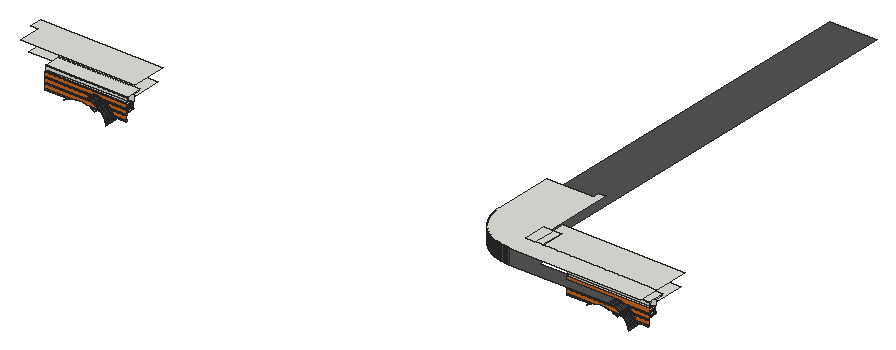
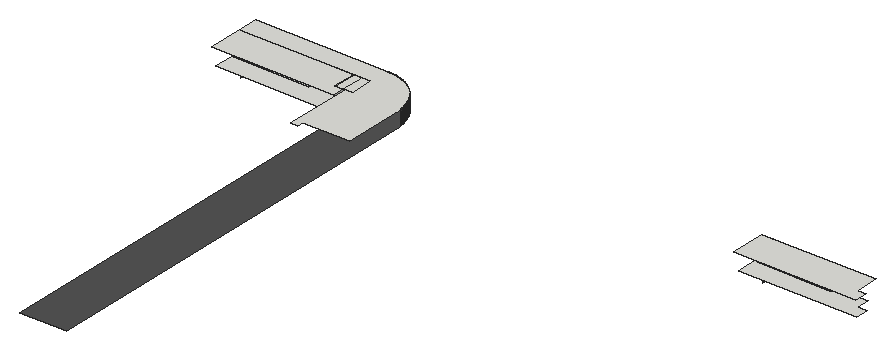
# SketchUp Ruby script. Lengths in inches.
U = 1.inch
M = Sketchup.active_model
def pt(a) = Geom::Point3d.new(a.map { |v| v * U })
def face(e, loops, mat)
  f = e.add_face(loops[0].map { |a| pt(a) })
  loops[1..].each { |l| e.add_face(l.map { |a| pt(a) }).erase! }
  f.material = f.back_material = mat if mat
  f
end
# faces: each face lists its corners as indices into pts; further lists are holes
def faces(e, pts, list, mat = nil) = list.each { |f| face(e, (f[0].is_a?(Array) ? f : [f]).map { |l| l.map { |i| pts[i] } }, mat) }
# xy, xz, yz: faces in a plane at the given z, y or x. An outline is a flat list of corners, or four numbers for a rectangle; further outlines are holes
def ring(l) = l.size == 4 ? [[l[0], l[1]], [l[2], l[1]], [l[2], l[3]], [l[0], l[3]]] : l.each_slice(2).to_a
def flat(e, list, mat, &to3) = list.each { |f| face(e, (f[0].is_a?(Array) ? f : [f]).map { |l| ring(l).map { |u, v| to3.(u, v) } }, mat) }
def xy(e, z, list, mat = nil) = flat(e, list, mat) { |x, y| [x, y, z] }
def xz(e, y, list, mat = nil) = flat(e, list, mat) { |x, z| [x, y, z] }
def yz(e, x, list, mat = nil) = flat(e, list, mat) { |y, z| [x, y, z] }
def lines(e, pts, list) = list.each { |a, b| e.add_line(pt(pts[a]), pt(pts[b])) }
# prism: a flat outline (further loops are holes) pulled along v
def prism(e, loops, v, mat = nil)
  f = face(e, loops, mat); d = Geom::Vector3d.new(v.map { |x| x * U })
  f.pushpull(f.normal.samedirection?(d) ? d.length : -d.length)
end
def box(e, o, s, mat = nil) = prism(e, [[o, [o[0] + s[0], o[1], o[2]], [o[0] + s[0], o[1] + s[1], o[2]], [o[0], o[1] + s[1], o[2]]]], [0, 0, s[2]], mat)
def at(x, y, z, deg = 0) = Geom::Transformation.translation(pt([x, y, z])) * Geom::Transformation.rotation(ORIGIN, Z_AXIS, deg.degrees)
def axes(o, x, y, z) = Geom::Transformation.new([*x, 0, *y, 0, *z, 0, *pt(o).to_a, 1])
def part(name) = M.definitions.add(name)
# library, detail: a bought-in or finely detailed component or shape, given as its bounding box
def library(name, o, s) = part(name).tap { |d| box(d.entities, o, s) }
def detail(e, o, s) = box(e.add_group.entities, o, s)
def put(e, d, t, mat = nil) = e.add_instance(d, t).tap { |i| i.material = mat if mat }
def group(e, t, mat = nil) = e.add_group.tap { |g| g.transformation = t; g.material = mat if mat }.entities
root = M.entities
M.materials.add("[0041_Chocolate]").color = [210, 105, 30]
M.materials.add("[Color M06]").color = [84, 84, 84]
xy(root,385.02,[[1547.71,280.47,1577.2,281.47],[1605.02,280.47,1649.14,281.47],[2198.21,280.47,2227.7,281.47],[2255.52,280.47,2299.64,281.47]],"[0041_Chocolate]")
xy(root,386.9375,[[1547.71,280.47,1582.17,281.47],[1600.06,280.47,1649.14,281.47],[2198.21,280.47,2232.67,281.47],[2250.56,280.47,2299.64,281.47]],"[0041_Chocolate]")
xy(root,391.89,[[1547.71,280.47,1649.14,281.47],[2198.21,280.47,2299.64,281.47]],"[0041_Chocolate]")
xy(root,393.8125,[[1547.71,280.47,1649.14,281.47],[2198.21,280.47,2299.64,281.47]],"[0041_Chocolate]")
xy(root,395.26,[[1547.71,302.46,1626.96,310.27],[2198.21,302.46,2277.46,310.27]])
xy(root,398.77,[[1547.71,280.47,1649.14,281.47],[2198.21,280.47,2299.64,281.47]],"[0041_Chocolate]")
xy(root,400.6875,[[1547.71,280.47,1649.14,281.47],[2198.21,280.47,2299.64,281.47]],"[0041_Chocolate]")
xy(root,402.64,[[1547.71,300.33,1608.92,302.46],[2198.21,300.33,2259.42,302.46],[1640.52,302.46,1643.23,302.46,1643.23,337.5625,1496.21,337.5625,1496.21,321.34,1507.74,321.34,1507.74,305.58,1547.71,305.58,1547.71,312.8125,1640.52,312.8125],[1547.71,302.46,1640.52,312.8125],[2291.02,302.46,2293.73,302.46,2293.73,337.5625,2146.71,337.5625,2146.71,321.34,2158.24,321.34,2158.24,305.58,2198.21,305.58,2198.21,312.8125,2291.02,312.8125],
  [2198.21,302.46,2291.02,312.8125],[2137,305.58,2146.71,312.8125],[2146.71,305.58,2158.24,312.8125],[2137,312.8125,2146.71,321.34]])
xy(root,402.64,[[2135.95,267.75,2134.46,267.77,2132.97,267.83,2131.49,267.93,2130.01,268.0625,2128.53,268.24,2127.05,268.45,2125.59,268.7,2124.125,268.99,2122.67,269.32,2121.23,269.6875,2119.8,270.09,2118.375,270.53,2116.96,271.01,2115.57,271.53,2114.18,272.08,2112.8125,272.67,2111.46,273.29,2110.125,273.95,2108.81,274.64,2107.51,275.37,2106.23,276.13,2104.97,276.93,2103.73,277.75,2102.51,278.61,2101.32,279.51,2100.15,280.43,2099.01,281.38,2097.89,282.36,2096.79,283.37,2095.73,284.41,2094.6875,285.48,2093.68,286.57,2092.69,287.69,2091.74,288.84,2090.82,290.01,2089.93,291.2,2089.07,292.42,2088.24,293.65,2087.45,294.91,2086.6875,296.19,2085.96,297.49,2085.27,298.8125,2084.61,300.15,2083.98,301.5,2083.4,302.87,2082.84,304.25,2082.33,305.65,2081.85,307.06,2081.41,308.48,2081,309.91,2080.64,311.36,2080.31,312.81,2080.02,314.27,2079.77,315.74,2079.55,317.21,2079.375,318.69,2079.24,320.17,2079.14,321.66,2079.08,323.15,2079.07,324.64,2079.07,838.14,2137,838.14,2137,305.58,2158.24,305.58,2158.24,287.95,2198.21,287.95,2198.21,300.33,2259.42,300.33,2259.42,267.75]],"[Color M06]")
xy(root,405.64,[[1547.71,280.47,1649.14,281.47],[2198.21,280.47,2299.64,281.47]],"[0041_Chocolate]")
xy(root,411.82,[[1547.71,281.47,1649.14,302.46],[2198.21,281.47,2299.64,302.46]])
xy(root,421.25,[[2135.95,267.75,2300.52,267.75,2300.52,292.45,2137,292.45,2137,321.34,2145.53,321.34,2145.53,406.38,2137,406.38,2137,397.86,2079.07,397.86,2079.07,324.64,2079.08,323.15,2079.14,321.66,2079.24,320.17,2079.375,318.69,2079.55,317.21,2079.77,315.74,2080.02,314.27,2080.31,312.81,2080.64,311.36,2081,309.91,2081.41,308.48,2081.85,307.06,2082.33,305.65,2082.84,304.25,2083.4,302.87,2083.98,301.5,2084.61,300.15,2085.27,298.8125,2085.96,297.49,2086.6875,296.19,2087.45,294.91,2088.24,293.65,2089.07,292.42,2089.93,291.2,2090.82,290.01,2091.74,288.84,2092.69,287.69,2093.68,286.57,2094.6875,285.48,2095.73,284.41,2096.79,283.37,2097.89,282.36,2099.01,281.38,2100.15,280.43,2101.32,279.51,2102.51,278.61,2103.73,277.75,2104.97,276.93,2106.23,276.13,2107.51,275.37,2108.81,274.64,2110.125,273.95,2111.46,273.29,2112.8125,272.67,2114.18,272.08,2115.57,271.53,2116.96,271.01,2118.375,270.53,2119.8,270.09,2121.23,269.6875,2122.67,269.32,2124.125,268.99,2125.59,268.7,2127.05,268.45,2128.53,268.24,2130.01,268.0625,2131.49,267.93,2132.97,267.83,2134.46,267.77],[1507.74,292.45,1650.02,292.45,1650.02,336.27,1498.09,336.27,1498.09,321.34,1507.74,321.34],[2137,292.45,2148.59,321.34],[2148.59,292.45,2158.24,321.34],[2158.24,292.45,2300.52,292.45,2300.52,336.27,2148.59,336.27,2148.59,321.34,2158.24,321.34]])
xz(root,280.47,[[1547.71,386.9375,1582.17,386.9375,1587,388.23,1595.19,388.24,1600.06,386.9375,1649.14,386.9375,1649.14,391.89,1547.71,391.89],[2198.21,386.9375,2232.67,386.9375,2237.5,388.23,2245.69,388.24,2250.56,386.9375,2299.64,386.9375,2299.64,391.89,2198.21,391.89],[1547.71,393.8125,1649.14,398.77],[2198.21,393.8125,2299.64,398.77],[1547.71,400.6875,1649.14,405.64],
  [2198.21,400.6875,2299.64,405.64]],"[0041_Chocolate]")
xz(root,281.47,[[1547.71,405.64,1649.14,407.5625],[2198.21,405.64,2299.64,407.5625],[1547.71,407.5625,1649.14,411.82],[2198.21,407.5625,2299.64,411.82],[1547.71,411.82,1649.14,412.52],
  [2198.21,411.82,2299.64,412.52]])
xz(root,281.47,[[1547.71,385.02,1577.2,385.02,1579.1,386.11,1582.17,386.9375,1547.71,386.9375],[1605.02,385.02,1649.14,385.02,1649.14,386.9375,1600.06,386.9375,1603.1,386.125],[2198.21,385.02,2227.7,385.02,2229.6,386.11,2232.67,386.9375,2198.21,386.9375],[2255.52,385.02,2299.64,385.02,2299.64,386.9375,2250.56,386.9375,2253.6,386.125],[1547.71,391.89,1649.14,393.8125],
  [2198.21,391.89,2299.64,393.8125],[1547.71,398.77,1649.14,400.6875],[2198.21,398.77,2299.64,400.6875]],"[0041_Chocolate]")
xz(root,302.46,[[1547.71,395.26,1626.96,395.26,1626.65,395.5625,1626.16,396.02,1625.65,396.46,1625.13,396.89,1624.6,397.3125,1624.06,397.72,1623.51,398.1,1622.95,398.48,1622.38,398.84,1621.8,399.18,1621.21,399.51,1620.61,399.83,1620.01,400.125,1619.4,400.41,1618.78,400.67,1618.15,400.92,1617.52,401.16,1616.88,401.375,1616.24,401.57,1615.59,401.76,1614.93,401.92,1614.27,402.07,1613.61,402.2,1612.95,402.32,1612.28,402.41,1611.61,402.49,1610.94,402.56,1610.27,402.6,1609.59,402.625,1608.92,402.64,1547.71,402.64],[1626.96,395.26,1634.68,395.26,1634.68,402.64,1608.92,402.64,1609.59,402.625,1610.27,402.6,1610.94,402.56,1611.61,402.49,1612.28,402.41,1612.95,402.32,1613.61,402.2,1614.27,402.07,1614.93,401.92,1615.59,401.76,1616.24,401.57,1616.88,401.375,1617.52,401.16,1618.15,400.92,1618.78,400.67,1619.4,400.41,1620.01,400.125,1620.61,399.83,1621.21,399.51,1621.8,399.18,1622.38,398.84,1622.95,398.48,1623.51,398.1,1624.06,397.72,1624.6,397.3125,1625.13,396.89,1625.65,396.46,1626.16,396.02,1626.65,395.5625],[1634.68,395.26,1640.52,402.64],[2198.21,395.26,2277.46,395.26,2277.15,395.5625,2276.66,396.02,2276.15,396.46,2275.63,396.89,2275.1,397.3125,2274.56,397.72,2274.01,398.1,2273.45,398.48,2272.88,398.84,2272.3,399.18,2271.71,399.51,2271.11,399.83,2270.51,400.125,2269.9,400.41,2269.28,400.67,2268.65,400.92,2268.02,401.16,2267.38,401.375,2266.74,401.57,2266.09,401.76,2265.43,401.92,2264.77,402.07,2264.11,402.2,2263.45,402.32,2262.78,402.41,2262.11,402.49,2261.44,402.56,2260.77,402.6,2260.09,402.625,2259.42,402.64,2198.21,402.64],[2277.46,395.26,2285.18,395.26,2285.18,402.64,2259.42,402.64,2260.09,402.625,2260.77,402.6,2261.44,402.56,2262.11,402.49,2262.78,402.41,2263.45,402.32,2264.11,402.2,2264.77,402.07,2265.43,401.92,2266.09,401.76,2266.74,401.57,2267.38,401.375,2268.02,401.16,2268.65,400.92,2269.28,400.67,2269.9,400.41,2270.51,400.125,2271.11,399.83,2271.71,399.51,2272.3,399.18,2272.88,398.84,2273.45,398.48,2274.01,398.1,2274.56,397.72,2275.1,397.3125,2275.63,396.89,2276.15,396.46,2276.66,396.02,2277.15,395.5625],
  [2285.18,395.26,2291.02,402.64],[1547.71,402.64,1634.68,411.82],[2198.21,402.64,2285.18,411.82]])
yz(root,1547.71,[[300.33,395.26,302.46,402.64],[302.46,395.26,305.58,402.64]])
yz(root,2158.24,[[292.45,402.64,321.34,421.25]])
yz(root,2198.21,[[300.33,395.26,302.46,402.64],[302.46,395.26,305.58,402.64]])
p = [[1634.25,267.75,381.57],[1634.25,302.46,381.57],[1634.36,302.46,380.9],[1634.36,267.75,380.9],[2284.75,267.75,381.57],[2284.75,302.46,381.57],
  [2284.86,302.46,380.9],[2284.86,267.75,380.9],[1634.36,310.27,380.9],[1634.25,310.27,381.57],[2284.86,310.27,380.9],[2284.75,310.27,381.57],
  [1634.12,267.75,382.23],[1634.12,302.46,382.23],[2284.62,267.75,382.23],[2284.62,302.46,382.23],[1634.12,310.27,382.23],[2284.62,310.27,382.23],
  [1577.2,295.65,385.02],[1577.2,281.47,385.02],[1577.2,280.47,385.02],[1572.01,280.47,382.01],[1572.01,295.65,382.01],[1610.19,295.65,382.03],
  [1610.19,280.47,382.03],[1605.02,280.47,385.02],[1605.02,281.47,385.02],[1605.02,295.65,385.02],[2227.7,295.65,385.02],[2227.7,281.47,385.02],
  [2227.7,280.47,385.02],[2222.51,280.47,382.01],[2222.51,295.65,382.01],[2260.69,295.65,382.03],[2260.69,280.47,382.03],[2255.52,280.47,385.02],
  [2255.52,281.47,385.02],[2255.52,295.65,385.02],[1633.97,267.75,382.89],[1633.97,302.46,382.89],[2284.47,267.75,382.89],[2284.47,302.46,382.89],
  [1633.97,310.27,382.89],[2284.47,310.27,382.89],[1633.8,267.75,383.54],[1633.8,302.46,383.54],[2284.3,267.75,383.54],[2284.3,302.46,383.54],
  [1633.8,310.27,383.54],[2284.3,310.27,383.54],[1633.62,267.75,384.19],[1633.62,302.46,384.19],[1633.78,302.46,383.64],[2284.12,267.75,384.19],
  [2284.12,302.46,384.19],[2284.28,302.46,383.64],[1633.78,310.27,383.64],[2284.28,310.27,383.64],[1633.62,310.27,384.19],[2284.12,310.27,384.19],
  [1633.42,267.75,384.84],[1633.42,302.46,384.84],[2283.92,267.75,384.84],[2283.92,302.46,384.84],[1633.42,310.27,384.84],[2283.92,310.27,384.84],
  [1633.2,267.75,385.47],[1633.2,302.46,385.47],[2283.7,267.75,385.47],[2283.7,302.46,385.47],[1633.2,310.27,385.47],[2283.7,310.27,385.47],
  [1579.1,281.47,386.11],[1579.1,295.65,386.11],[1603.1,281.47,386.125],[1603.1,295.65,386.125],[2229.6,281.47,386.11],[2229.6,295.65,386.11],
  [2253.6,281.47,386.125],[2253.6,295.65,386.125],[1632.97,267.75,386.11],[1632.97,302.46,386.11],[1633.1,302.46,385.76],[2283.47,267.75,386.11],
  [2283.47,302.46,386.11],[2283.6,302.46,385.76],[1633.1,310.27,385.76],[2283.6,310.27,385.76],[1632.97,310.27,386.11],[2283.47,310.27,386.11],
  [1632.72,267.75,386.73],[1632.72,302.46,386.73],[2283.22,267.75,386.73],[2283.22,302.46,386.73],[1582.17,281.47,386.9375],[1582.17,295.65,386.9375],
  [1600.06,281.47,386.9375],[1600.06,295.65,386.9375],[2232.67,281.47,386.9375],[2232.67,295.65,386.9375],[2250.56,281.47,386.9375],[2250.56,295.65,386.9375],
  [1632.72,310.27,386.73],[2283.22,310.27,386.73],[1632.45,267.75,387.35],[1632.45,302.46,387.35],[2282.95,267.75,387.35],[2282.95,302.46,387.35],
  [1632.45,310.27,387.35],[2282.95,310.27,387.35],[1587,295.65,388.23],[1587,280.47,388.23],[1582.17,280.47,386.9375],[1600.06,280.47,386.9375],
  [1595.19,280.47,388.24],[1595.19,295.65,388.24],[2237.5,295.65,388.23],[2237.5,280.47,388.23],[2232.67,280.47,386.9375],[2250.56,280.47,386.9375],
  [2245.69,280.47,388.24],[2245.69,295.65,388.24],[1632.17,267.75,387.96],[1632.17,302.46,387.96],[2282.67,267.75,387.96],[2282.67,302.46,387.96],
  [1632.17,310.27,387.96],[2282.67,310.27,387.96],[1631.87,267.75,388.57],[1631.87,302.46,388.57],[2282.37,267.75,388.57],[2282.37,302.46,388.57],
  [1631.87,310.27,388.57],[2282.37,310.27,388.57],[1631.56,267.75,389.17],[1631.56,302.46,389.17],[2282.06,267.75,389.17],[2282.06,302.46,389.17],
  [1631.56,310.27,389.17],[2282.06,310.27,389.17],[1631.23,267.75,389.76],[1631.23,302.46,389.76],[2281.73,267.75,389.76],[2281.73,302.46,389.76],
  [1631.23,310.27,389.76],[2281.73,310.27,389.76],[1630.88,267.75,390.33],[1630.88,302.46,390.33],[2281.38,267.75,390.33],[2281.38,302.46,390.33],
  [1630.88,310.27,390.33],[2281.38,310.27,390.33],[1630.52,267.75,390.9],[1630.52,302.46,390.9],[2281.02,267.75,390.9],[2281.02,302.46,390.9],
  [1630.52,310.27,390.9],[2281.02,310.27,390.9],[1630.15,267.75,391.47],[1630.15,302.46,391.47],[2280.65,267.75,391.47],[2280.65,302.46,391.47],
  [1630.15,310.27,391.47],[2280.65,310.27,391.47],[1629.76,267.75,392.02],[1629.76,302.46,392.02],[2280.26,267.75,392.02],[2280.26,302.46,392.02],
  [1629.76,310.27,392.02],[2280.26,310.27,392.02],[1629.36,267.75,392.56],[1629.36,302.46,392.56],[2279.86,267.75,392.56],[2279.86,302.46,392.56],
  [1629.36,310.27,392.56],[2279.86,310.27,392.56],[1628.9375,267.75,393.09],[1628.9375,302.46,393.09],[2279.4375,267.75,393.09],[2279.4375,302.46,393.09],
  [1628.9375,310.27,393.09],[2279.4375,310.27,393.09],[1628.51,267.75,393.6],[1628.51,302.46,393.6],[1628.9,302.46,393.14],[2279.01,267.75,393.6],
  [2279.01,302.46,393.6],[2279.4,302.46,393.14],[1628.9,310.27,393.14],[1628.51,310.27,393.6],[2279.4,310.27,393.14],[2279.01,310.27,393.6],
  [1628.0625,267.75,394.11],[1628.0625,302.46,394.11],[2278.5625,267.75,394.11],[2278.5625,302.46,394.11],[1628.0625,310.27,394.11],[2278.5625,310.27,394.11],
  [1627.6,267.75,394.61],[1627.6,302.46,394.61],[2278.1,267.75,394.61],[2278.1,302.46,394.61],[1627.6,310.27,394.61],[2278.1,310.27,394.61],
  [1627.13,267.75,395.09],[1627.13,302.46,395.09],[2277.63,267.75,395.09],[2277.63,302.46,395.09],[1627.13,310.27,395.09],[2277.63,310.27,395.09],
  [1626.65,267.75,395.5625],[1626.65,300.33,395.5625],[1626.96,300.33,395.26],[1626.96,302.46,395.26],[2277.15,267.75,395.5625],[2277.15,300.33,395.5625],
  [2277.46,300.33,395.26],[2277.46,302.46,395.26],[1626.96,310.27,395.26],[2277.46,310.27,395.26],[1626.65,302.46,395.5625],[2277.15,302.46,395.5625],
  [1626.16,267.75,396.02],[1626.16,300.33,396.02],[2276.66,267.75,396.02],[2276.66,300.33,396.02],[1626.16,302.46,396.02],[2276.66,302.46,396.02],
  [1625.65,267.75,396.46],[1625.65,300.33,396.46],[2276.15,267.75,396.46],[2276.15,300.33,396.46],[1625.65,302.46,396.46],[2276.15,302.46,396.46],
  [1625.13,267.75,396.89],[1625.13,300.33,396.89],[2275.63,267.75,396.89],[2275.63,300.33,396.89],[1625.13,302.46,396.89],[2275.63,302.46,396.89],
  [1624.6,267.75,397.3125],[1624.6,300.33,397.3125],[2275.1,267.75,397.3125],[2275.1,300.33,397.3125],[1624.6,302.46,397.3125],[2275.1,302.46,397.3125],
  [1624.06,267.75,397.72],[1624.06,300.33,397.72],[2274.56,267.75,397.72],[2274.56,300.33,397.72],[1624.06,302.46,397.72],[2274.56,302.46,397.72],
  [1623.51,267.75,398.1],[1623.51,300.33,398.1],[2274.01,267.75,398.1],[2274.01,300.33,398.1],[1623.51,302.46,398.1],[2274.01,302.46,398.1],
  [1622.95,267.75,398.48],[1622.95,300.33,398.48],[2273.45,267.75,398.48],[2273.45,300.33,398.48],[1622.95,302.46,398.48],[2273.45,302.46,398.48],
  [1622.38,267.75,398.84],[1622.38,300.33,398.84],[2272.88,267.75,398.84],[2272.88,300.33,398.84],[1622.38,302.46,398.84],[2272.88,302.46,398.84],
  [1621.8,267.75,399.18],[1621.8,300.33,399.18],[2272.3,267.75,399.18],[2272.3,300.33,399.18],[1621.8,302.46,399.18],[2272.3,302.46,399.18],
  [1621.21,267.75,399.51],[1621.21,300.33,399.51],[2271.71,267.75,399.51],[2271.71,300.33,399.51],[1621.21,302.46,399.51],[2271.71,302.46,399.51],
  [1620.61,267.75,399.83],[1620.61,300.33,399.83],[2271.11,267.75,399.83],[2271.11,300.33,399.83],[1620.61,302.46,399.83],[2271.11,302.46,399.83],
  [1620.01,267.75,400.125],[1620.01,300.33,400.125],[2270.51,267.75,400.125],[2270.51,300.33,400.125],[1620.01,302.46,400.125],[2270.51,302.46,400.125],
  [1619.4,267.75,400.41],[1619.4,300.33,400.41],[2269.9,267.75,400.41],[2269.9,300.33,400.41],[1619.4,302.46,400.41],[2269.9,302.46,400.41],
  [1618.78,267.75,400.67],[1618.78,300.33,400.67],[2269.28,267.75,400.67],[2269.28,300.33,400.67],[1618.78,302.46,400.67],[2269.28,302.46,400.67],
  [1618.15,267.75,400.92],[1618.15,300.33,400.92],[2268.65,267.75,400.92],[2268.65,300.33,400.92],[1618.15,302.46,400.92],[2268.65,302.46,400.92],
  [1617.52,267.75,401.16],[1617.52,300.33,401.16],[2268.02,267.75,401.16],[2268.02,300.33,401.16],[1617.52,302.46,401.16],[2268.02,302.46,401.16],
  [1616.88,267.75,401.375],[1616.88,300.33,401.375],[2267.38,267.75,401.375],[2267.38,300.33,401.375],[1616.88,302.46,401.375],[2267.38,302.46,401.375],
  [1616.24,267.75,401.57],[1616.24,300.33,401.57],[2266.74,267.75,401.57],[2266.74,300.33,401.57],[1616.24,302.46,401.57],[2266.74,302.46,401.57],
  [1615.59,267.75,401.76],[1615.59,300.33,401.76],[2266.09,267.75,401.76],[2266.09,300.33,401.76],[1615.59,302.46,401.76],[2266.09,302.46,401.76],
  [1614.93,267.75,401.92],[1614.93,300.33,401.92],[2265.43,267.75,401.92],[2265.43,300.33,401.92],[1614.93,302.46,401.92],[2265.43,302.46,401.92],
  [1614.27,267.75,402.07],[1614.27,300.33,402.07],[2264.77,267.75,402.07],[2264.77,300.33,402.07],[1614.27,302.46,402.07],[2264.77,302.46,402.07],
  [1613.61,267.75,402.2],[1613.61,300.33,402.2],[2264.11,267.75,402.2],[2264.11,300.33,402.2],[1613.61,302.46,402.2],[2264.11,302.46,402.2],
  [1612.95,267.75,402.32],[1612.95,300.33,402.32],[2263.45,267.75,402.32],[2263.45,300.33,402.32],[1612.95,302.46,402.32],[2263.45,302.46,402.32],
  [1612.28,267.75,402.41],[1612.28,300.33,402.41],[2262.78,267.75,402.41],[2262.78,300.33,402.41],[1612.28,302.46,402.41],[2262.78,302.46,402.41],
  [1611.61,267.75,402.49],[1611.61,300.33,402.49],[2262.11,267.75,402.49],[2262.11,300.33,402.49],[1611.61,302.46,402.49],[2262.11,302.46,402.49],
  [1610.94,267.75,402.56],[1610.94,300.33,402.56],[2261.44,267.75,402.56],[2261.44,300.33,402.56],[1610.94,302.46,402.56],[2261.44,302.46,402.56],
  [1608.92,267.75,402.64],[1608.92,300.33,402.64],[1609.59,300.33,402.625],[1609.59,267.75,402.625],[1610.27,300.33,402.6],[1610.27,267.75,402.6],
  [2132.97,267.83,421.25],[2131.49,267.93,421.25],[2131.49,267.93,402.64],[2132.97,267.83,402.64],[2134.46,267.77,421.25],[2134.46,267.77,402.64],
  [2135.95,267.75,421.25],[2135.95,267.75,402.64],[2259.42,267.75,402.64],[2259.42,300.33,402.64],[2260.09,300.33,402.625],[2260.09,267.75,402.625],
  [2260.77,300.33,402.6],[2260.77,267.75,402.6],[2130.01,268.0625,421.25],[2130.01,268.0625,402.64],[2128.53,268.24,421.25],[2128.53,268.24,402.64],
  [2127.05,268.45,421.25],[2127.05,268.45,402.64],[2125.59,268.7,421.25],[2125.59,268.7,402.64],[2124.125,268.99,421.25],[2124.125,268.99,402.64],
  [2122.67,269.32,421.25],[2122.67,269.32,402.64],[2121.23,269.6875,421.25],[2121.23,269.6875,402.64],[2119.8,270.09,421.25],[2119.8,270.09,402.64],
  [2118.375,270.53,421.25],[2118.375,270.53,402.64],[2116.96,271.01,421.25],[2116.96,271.01,402.64],[2115.57,271.53,421.25],[2115.57,271.53,402.64],
  [2114.18,272.08,421.25],[2114.18,272.08,402.64],[2112.8125,272.67,421.25],[2112.8125,272.67,402.64],[2111.46,273.29,421.25],[2111.46,273.29,402.64],
  [2110.125,273.95,421.25],[2110.125,273.95,402.64],[2108.81,274.64,421.25],[2108.81,274.64,402.64],[2107.51,275.37,421.25],[2107.51,275.37,402.64],
  [2106.23,276.13,421.25],[2106.23,276.13,402.64],[2104.97,276.93,421.25],[2104.97,276.93,402.64],[2103.73,277.75,421.25],[2103.73,277.75,402.64],
  [2102.51,278.61,421.25],[2102.51,278.61,402.64],[2101.32,279.51,421.25],[2101.32,279.51,402.64],[2100.15,280.43,421.25],[2100.15,280.43,402.64],
  [2099.01,281.38,421.25],[2099.01,281.38,402.64],[2097.89,282.36,421.25],[2097.89,282.36,402.64],[2096.79,283.37,421.25],[2096.79,283.37,402.64],
  [2095.73,284.41,421.25],[2095.73,284.41,402.64],[2094.6875,285.48,421.25],[2094.6875,285.48,402.64],[2093.68,286.57,421.25],[2093.68,286.57,402.64],
  [2092.69,287.69,421.25],[2092.69,287.69,402.64],[2091.74,288.84,421.25],[2091.74,288.84,402.64],[2090.82,290.01,421.25],[2090.82,290.01,402.64],
  [2089.93,291.2,421.25],[2089.93,291.2,402.64],[2089.07,292.42,421.25],[2089.07,292.42,402.64],[2088.24,293.65,421.25],[2088.24,293.65,402.64],
  [2087.45,294.91,421.25],[2087.45,294.91,402.64],[2086.6875,296.19,421.25],[2086.6875,296.19,402.64],[2085.96,297.49,421.25],[2085.96,297.49,402.64],
  [2085.27,298.8125,421.25],[2085.27,298.8125,402.64],[2084.61,300.15,421.25],[2084.61,300.15,402.64],[2083.98,301.5,421.25],[2083.98,301.5,402.64],
  [1608.92,302.46,402.64],[1609.59,302.46,402.625],[1610.27,302.46,402.6],[2259.42,302.46,402.64],[2260.09,302.46,402.625],[2260.77,302.46,402.6],
  [2083.4,302.87,421.25],[2083.4,302.87,402.64],[2082.84,304.25,421.25],[2082.84,304.25,402.64],[2082.33,305.65,421.25],[2082.33,305.65,402.64],
  [2081.85,307.06,421.25],[2081.85,307.06,402.64],[2081.41,308.48,421.25],[2081.41,308.48,402.64],[2081,309.91,421.25],[2081,309.91,402.64],
  [2080.64,311.36,421.25],[2080.64,311.36,402.64],[2080.31,312.81,421.25],[2080.31,312.81,402.64],[2080.02,314.27,421.25],[2080.02,314.27,402.64],
  [2079.77,315.74,421.25],[2079.77,315.74,402.64],[2079.55,317.21,421.25],[2079.55,317.21,402.64]]
faces(root,p,[[0,1,2,3],[4,5,6,7],[12,13,1,0],[14,15,5,4],[38,39,13,12],[40,41,15,14],[44,45,39,38],[46,47,41,40],
  [50,51,52,45,44],[53,54,55,47,46],[60,61,51,50],[62,63,54,53],[66,67,61,60],[68,69,63,62],[80,81,82,67,66],[83,84,85,69,68],
  [90,91,81,80],[92,93,84,83],[104,105,91,90],[106,107,93,92],[122,123,105,104],[124,125,107,106],[128,129,123,122],[130,131,125,124],
  [134,135,129,128],[136,137,131,130],[140,141,135,134],[142,143,137,136],[146,147,141,140],[148,149,143,142],[152,153,147,146],[154,155,149,148],
  [158,159,153,152],[160,161,155,154],[164,165,159,158],[166,167,161,160],[170,171,165,164],[172,173,167,166],[176,177,171,170],[178,179,173,172],
  [182,183,184,177,176],[185,186,187,179,178],[192,193,183,182],[194,195,186,185],[198,199,193,192],[200,201,195,194],[204,205,199,198],[206,207,201,200],
  [210,211,212,213,205,204],[214,215,216,217,207,206],[222,223,211,210],[224,225,215,214],[228,229,223,222],[230,231,225,224],[234,235,229,228],[236,237,231,230],
  [240,241,235,234],[242,243,237,236],[246,247,241,240],[248,249,243,242],[252,253,247,246],[254,255,249,248],[258,259,253,252],[260,261,255,254],
  [264,265,259,258],[266,267,261,260],[270,271,265,264],[272,273,267,266],[276,277,271,270],[278,279,273,272],[282,283,277,276],[284,285,279,278],
  [288,289,283,282],[290,291,285,284],[294,295,289,288],[296,297,291,290],[300,301,295,294],[302,303,297,296],[306,307,301,300],[308,309,303,302],
  [312,313,307,306],[314,315,309,308],[318,319,313,312],[320,321,315,314],[324,325,319,318],[326,327,321,320],[330,331,325,324],[332,333,327,326],
  [336,337,331,330],[338,339,333,332],[342,343,337,336],[344,345,339,338],[348,349,343,342],[350,351,345,344],[354,355,349,348],[356,357,351,350],
  [360,361,355,354],[362,363,357,356],[366,367,361,360],[368,369,363,362],[372,373,367,366],[374,375,369,368],[378,379,380,381],[381,380,382,383],
  [383,382,373,372],[384,385,386,387],[388,384,387,389],[390,388,389,391],[392,393,394,395],[395,394,396,397],[397,396,375,374],[385,398,399,386],
  [398,400,401,399],[400,402,403,401],[402,404,405,403],[404,406,407,405],[406,408,409,407],[408,410,411,409],[410,412,413,411],[412,414,415,413],
  [414,416,417,415],[416,418,419,417],[418,420,421,419],[420,422,423,421],[422,424,425,423],[424,426,427,425],[426,428,429,427],[428,430,431,429],
  [430,432,433,431],[432,434,435,433],[434,436,437,435],[436,438,439,437],[438,440,441,439],[440,442,443,441],[442,444,445,443],[444,446,447,445],
  [446,448,449,447],[448,450,451,449],[450,452,453,451],[452,454,455,453],[454,456,457,455],[456,458,459,457],[458,460,461,459],[460,462,463,461],
  [462,464,465,463],[464,466,467,465],[466,468,469,467],[468,470,471,469],[470,472,473,471],[472,474,475,473],[474,476,477,475],[476,478,479,477],
  [478,486,487,479],[486,488,489,487],[488,490,491,489],[490,492,493,491],[492,494,495,493],[494,496,497,495],[496,498,499,497],[498,500,501,499],
  [500,502,503,501],[502,504,505,503],[504,506,507,505]],"[Color M06]")
faces(root,p,[[1,2,8,9],[5,6,10,11],[13,1,9,16],[15,5,11,17],[18,19,20,21,22],[23,24,25,26,27],[28,29,30,31,32],[33,34,35,36,37],
  [39,13,16,42],[41,15,17,43],[45,39,42,48],[47,41,43,49],[52,45,48,56],[55,47,49,57],[51,52,56,58],[54,55,57,59],
  [61,51,58,64],[63,54,59,65],[67,61,64,70],[69,63,65,71],[72,19,18,73],[26,74,75,27],[76,29,28,77],[36,78,79,37],
  [82,67,70,86],[85,69,71,87],[81,82,86,88],[84,85,87,89],[94,72,73,95],[74,96,97,75],[98,76,77,99],[78,100,101,79],
  [91,81,88,102],[93,84,89,103],[105,91,102,108],[107,93,103,109],[110,111,112,94,95],[97,96,113,114,115],[116,117,118,98,99],[101,100,119,120,121],
  [123,105,108,126],[125,107,109,127],[129,123,126,132],[131,125,127,133],[115,114,111,110],[121,120,117,116],[135,129,132,138],[137,131,133,139],
  [141,135,138,144],[143,137,139,145],[147,141,144,150],[149,143,145,151],[153,147,150,156],[155,149,151,157],[159,153,156,162],[161,155,157,163],
  [165,159,162,168],[167,161,163,169],[171,165,168,174],[173,167,169,175],[177,171,174,180],[179,173,175,181],[183,184,188,189],[184,177,180,188],
  [186,187,190,191],[187,179,181,190],[193,183,189,196],[195,186,191,197],[199,193,196,202],[201,195,197,203],[205,199,202,208],[207,201,203,209],
  [213,205,208,218],[217,207,209,219],[220,213,212,211],[221,217,216,215],[226,220,211,223],[227,221,215,225],[232,226,223,229],[233,227,225,231],
  [238,232,229,235],[239,233,231,237],[244,238,235,241],[245,239,237,243],[250,244,241,247],[251,245,243,249],[256,250,247,253],[257,251,249,255],
  [262,256,253,259],[263,257,255,261],[268,262,259,265],[269,263,261,267],[274,268,265,271],[275,269,267,273],[280,274,271,277],[281,275,273,279],
  [286,280,277,283],[287,281,279,285],[292,286,283,289],[293,287,285,291],[298,292,289,295],[299,293,291,297],[304,298,295,301],[305,299,297,303],
  [310,304,301,307],[311,305,303,309],[316,310,307,313],[317,311,309,315],[322,316,313,319],[323,317,315,321],[328,322,319,325],[329,323,321,327],
  [334,328,325,331],[335,329,327,333],[340,334,331,337],[341,335,333,339],[346,340,337,343],[347,341,339,345],[352,346,343,349],[353,347,345,351],
  [358,352,349,355],[359,353,351,357],[364,358,355,361],[365,359,357,363],[370,364,361,367],[371,365,363,369],[376,370,367,373],[377,371,369,375],
  [480,481,380,379],[481,482,382,380],[482,376,373,382],[483,484,394,393],[484,485,396,394],[485,377,375,396]])
